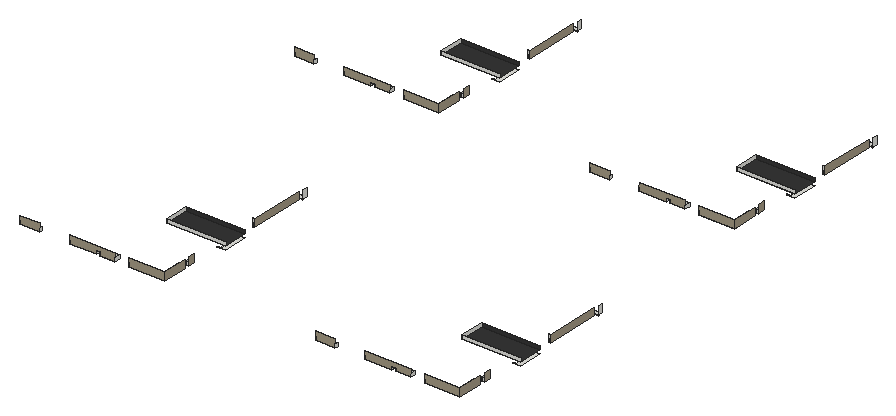
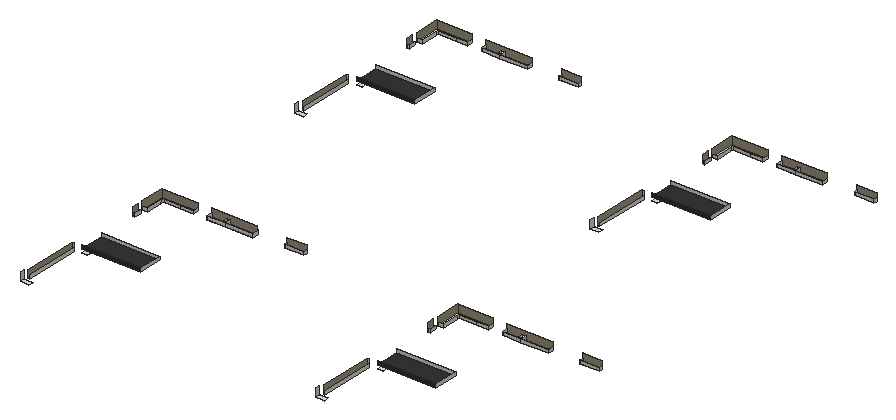
# SketchUp Ruby script. Lengths in inches.
U = 1.inch
M = Sketchup.active_model
def pt(a) = Geom::Point3d.new(a.map { |v| v * U })
def face(e, loops, mat)
  f = e.add_face(loops[0].map { |a| pt(a) })
  loops[1..].each { |l| e.add_face(l.map { |a| pt(a) }).erase! }
  f.material = f.back_material = mat if mat
  f
end
# faces: each face lists its corners as indices into pts; further lists are holes
def faces(e, pts, list, mat = nil) = list.each { |f| face(e, (f[0].is_a?(Array) ? f : [f]).map { |l| l.map { |i| pts[i] } }, mat) }
# xy, xz, yz: faces in a plane at the given z, y or x. An outline is a flat list of corners, or four numbers for a rectangle; further outlines are holes
def ring(l) = l.size == 4 ? [[l[0], l[1]], [l[2], l[1]], [l[2], l[3]], [l[0], l[3]]] : l.each_slice(2).to_a
def flat(e, list, mat, &to3) = list.each { |f| face(e, (f[0].is_a?(Array) ? f : [f]).map { |l| ring(l).map { |u, v| to3.(u, v) } }, mat) }
def xy(e, z, list, mat = nil) = flat(e, list, mat) { |x, y| [x, y, z] }
def xz(e, y, list, mat = nil) = flat(e, list, mat) { |x, z| [x, y, z] }
def yz(e, x, list, mat = nil) = flat(e, list, mat) { |y, z| [x, y, z] }
def lines(e, pts, list) = list.each { |a, b| e.add_line(pt(pts[a]), pt(pts[b])) }
# prism: a flat outline (further loops are holes) pulled along v
def prism(e, loops, v, mat = nil)
  f = face(e, loops, mat); d = Geom::Vector3d.new(v.map { |x| x * U })
  f.pushpull(f.normal.samedirection?(d) ? d.length : -d.length)
end
def box(e, o, s, mat = nil) = prism(e, [[o, [o[0] + s[0], o[1], o[2]], [o[0] + s[0], o[1] + s[1], o[2]], [o[0], o[1] + s[1], o[2]]]], [0, 0, s[2]], mat)
def at(x, y, z, deg = 0) = Geom::Transformation.translation(pt([x, y, z])) * Geom::Transformation.rotation(ORIGIN, Z_AXIS, deg.degrees)
def axes(o, x, y, z) = Geom::Transformation.new([*x, 0, *y, 0, *z, 0, *pt(o).to_a, 1])
def part(name) = M.definitions.add(name)
# library, detail: a bought-in or finely detailed component or shape, given as its bounding box
def library(name, o, s) = part(name).tap { |d| box(d.entities, o, s) }
def detail(e, o, s) = box(e.add_group.entities, o, s)
def put(e, d, t, mat = nil) = e.add_instance(d, t).tap { |i| i.material = mat if mat }
def group(e, t, mat = nil) = e.add_group.tap { |g| g.transformation = t; g.material = mat if mat }.entities
root = M.entities
M.materials.add("[Concrete Tile]").color = [165, 155, 133]
M.materials.add("[Slate Light Tile]").color = [54, 54, 54]
xy(root,88.32,[[879.125,2113.57,879.125,2115.31,892.3125,2115.31,892.3125,2213.62,913.875,2213.62,913.875,2113.57],[2097.3125,2113.57,2097.3125,2115.31,2110.5,2115.31,2110.5,2213.62,2132.0625,2213.62,2132.0625,2113.57],[890.875,2115.31,892.3125,2213.62],[2109.0625,2115.31,2110.5,2213.62],[879.125,3528.25,879.125,3530,892.3125,3530,892.3125,3628.31,913.875,3628.31,913.875,3528.25],
  [2097.3125,3528.25,2097.3125,3530,2110.5,3530,2110.5,3628.31,2132.0625,3628.31,2132.0625,3528.25],[890.875,3530,892.3125,3628.31],[2109.0625,3530,2110.5,3628.31]])
xy(root,103.85,[[671.25,2113.57,913.875,2213.62],[1889.4375,2113.57,2132.0625,2213.62],[671.25,3528.25,913.875,3628.31],[1889.4375,3528.25,2132.0625,3628.31]],"[Slate Light Tile]")
xy(root,112.625,[[319.53,1799.9375,399.88,1811.4375],[521.59,1799.9375,634.11,1822.9375],[647.8,1799.9375,647.8,1814.92,634.11,1814.92,634.11,1822.9375,709.87,1822.9375,709.87,1799.9375],[767.19,1799.9375,767.19,1822.9375,890.875,1822.9375,890.875,1902.66,913.875,1902.66,913.875,1799.9375],[1537.72,1799.9375,1618.07,1811.4375],
  [1739.78,1799.9375,1852.3,1822.9375],[1865.99,1799.9375,1865.99,1814.92,1852.3,1814.92,1852.3,1822.9375,1928.05,1822.9375,1928.05,1799.9375],[1985.38,1799.9375,1985.38,1822.9375,2109.0625,1822.9375,2109.0625,1902.66,2132.0625,1902.66,2132.0625,1799.9375],[902.375,1926.07,913.875,1953.7],[2120.5625,1926.07,2132.0625,1953.7],
  [913.875,2257.8125,921.125,2483.21],[2132.0625,2257.8125,2139.3125,2483.21],[890.875,2497.47,927.0625,2514.84],[2109.0625,2497.47,2145.25,2514.84],[319.53,3214.625,399.88,3226.125],
  [521.59,3214.625,634.11,3237.625],[647.8,3214.625,647.8,3229.61,634.11,3229.61,634.11,3237.625,709.87,3237.625,709.87,3214.625],[767.19,3214.625,767.19,3237.625,890.875,3237.625,890.875,3317.34,913.875,3317.34,913.875,3214.625],[1537.72,3214.625,1618.07,3226.125],[1739.78,3214.625,1852.3,3237.625],
  [1865.99,3214.625,1865.99,3229.61,1852.3,3229.61,1852.3,3237.625,1928.05,3237.625,1928.05,3214.625],[1985.38,3214.625,1985.38,3237.625,2109.0625,3237.625,2109.0625,3317.34,2132.0625,3317.34,2132.0625,3214.625],[902.375,3340.76,913.875,3368.39],[2120.5625,3340.76,2132.0625,3368.39],[913.875,3672.5,921.125,3897.9],
  [2132.0625,3672.5,2139.3125,3897.9],[890.875,3912.16,927.0625,3929.52],[2109.0625,3912.16,2145.25,3929.52]])
xz(root,1799.9375,[[319.53,112.625,399.88,145.375],[521.59,112.625,634.11,112.625,634.11,126,647.8,126,647.8,112.625,709.87,112.625,709.87,145.375,523.04,145.375,523.04,132,521.59,132],[767.19,112.625,913.875,145.375],[1537.72,112.625,1618.07,145.375],[1739.78,112.625,1852.3,112.625,1852.3,126,1865.99,126,1865.99,112.625,1928.05,112.625,1928.05,145.375,1741.23,145.375,1741.23,132,1739.78,132],
  [1985.38,112.625,2132.0625,145.375]],"[Concrete Tile]")
xz(root,1811.4375,[[319.53,112.625,399.88,126],[1537.72,112.625,1618.07,126]])
xz(root,1814.92,[[634.11,112.625,647.8,124.32],[1852.3,112.625,1865.99,124.32]])
xz(root,1822.9375,[[521.59,112.625,634.11,126],[634.11,112.625,709.87,126],[767.19,112.625,817,126],[817,112.625,890.875,126],[1739.78,112.625,1852.3,126],
  [1852.3,112.625,1928.05,126],[1985.38,112.625,2035.1875,126],[2035.1875,112.625,2109.0625,126]])
xz(root,1902.66,[[890.875,112.625,913.875,126],[2109.0625,112.625,2132.0625,126]])
xz(root,1926.07,[[902.375,112.625,913.875,126],[2120.5625,112.625,2132.0625,126]])
xz(root,1953.7,[[902.375,112.625,913.875,126],[2120.5625,112.625,2132.0625,126]])
xz(root,2113.57,[[671.25,103.85,913.875,117.41],[1889.4375,103.85,2132.0625,117.41]])
xz(root,2213.62,[[671.25,103.85,913.875,117.41],[1889.4375,103.85,2132.0625,117.41]],"[Slate Light Tile]")
xz(root,2257.8125,[[913.875,112.625,921.125,143.875],[2132.0625,112.625,2139.3125,143.875]])
xz(root,2497.47,[[921.125,110.625,921.125,112.625,927.0625,112.625,927.0625,143.875,927.75,143.875,927.75,110.625],[2139.3125,110.625,2139.3125,112.625,2145.25,112.625,2145.25,143.875,2145.9375,143.875,2145.9375,110.625]])
xz(root,3214.625,[[319.53,112.625,399.88,145.375],[521.59,112.625,634.11,112.625,634.11,126,647.8,126,647.8,112.625,709.87,112.625,709.87,145.375,523.04,145.375,523.04,132,521.59,132],[767.19,112.625,913.875,145.375],[1537.72,112.625,1618.07,145.375],[1739.78,112.625,1852.3,112.625,1852.3,126,1865.99,126,1865.99,112.625,1928.05,112.625,1928.05,145.375,1741.23,145.375,1741.23,132,1739.78,132],
  [1985.38,112.625,2132.0625,145.375]],"[Concrete Tile]")
xz(root,3226.125,[[319.53,112.625,399.88,126],[1537.72,112.625,1618.07,126]])
xz(root,3229.61,[[634.11,112.625,647.8,124.32],[1852.3,112.625,1865.99,124.32]])
xz(root,3237.625,[[521.59,112.625,634.11,126],[634.11,112.625,709.87,126],[767.19,112.625,817,126],[817,112.625,890.875,126],[1739.78,112.625,1852.3,126],
  [1852.3,112.625,1928.05,126],[1985.38,112.625,2035.1875,126],[2035.1875,112.625,2109.0625,126]])
xz(root,3317.34,[[890.875,112.625,913.875,126],[2109.0625,112.625,2132.0625,126]])
xz(root,3340.76,[[902.375,112.625,913.875,126],[2120.5625,112.625,2132.0625,126]])
xz(root,3368.39,[[902.375,112.625,913.875,126],[2120.5625,112.625,2132.0625,126]])
xz(root,3528.25,[[671.25,103.85,913.875,117.41],[1889.4375,103.85,2132.0625,117.41]])
xz(root,3628.31,[[671.25,103.85,913.875,117.41],[1889.4375,103.85,2132.0625,117.41]],"[Slate Light Tile]")
xz(root,3672.5,[[913.875,112.625,921.125,143.875],[2132.0625,112.625,2139.3125,143.875]])
xz(root,3912.16,[[921.125,110.625,921.125,112.625,927.0625,112.625,927.0625,143.875,927.75,143.875,927.75,110.625],[2139.3125,110.625,2139.3125,112.625,2145.25,112.625,2145.25,143.875,2145.9375,143.875,2145.9375,110.625]])
yz(root,319.53,[[1799.9375,112.625,1811.4375,126],[3214.625,112.625,3226.125,126]])
yz(root,399.88,[[1799.9375,112.625,1811.4375,126],[3214.625,112.625,3226.125,126]])
yz(root,521.59,[[1799.9375,112.625,1822.9375,126],[3214.625,112.625,3237.625,126]])
yz(root,634.11,[[1799.9375,112.625,1814.92,126],[3214.625,112.625,3229.61,126]])
yz(root,647.8,[[1799.9375,112.625,1814.92,126],[3214.625,112.625,3229.61,126]])
yz(root,671.25,[[2113.57,103.85,2213.62,117.41],[3528.25,103.85,3628.31,117.41]])
yz(root,709.87,[[1799.9375,112.625,1822.9375,126],[3214.625,112.625,3237.625,126]])
yz(root,767.19,[[1799.9375,112.625,1822.9375,126],[3214.625,112.625,3237.625,126]])
yz(root,890.875,[[1822.9375,112.625,1834.0625,126],[1834.0625,112.625,1902.66,126],[3237.625,112.625,3248.75,126],[3248.75,112.625,3317.34,126]])
yz(root,902.375,[[1926.07,112.625,1953.7,126],[3340.76,112.625,3368.39,126]])
yz(root,913.875,[[2257.8125,112.625,2483.21,126],[3672.5,112.625,3897.9,126]])
yz(root,913.875,[[1799.9375,112.625,1902.66,145.375],[1926.07,112.625,1953.7,145.375],[3214.625,112.625,3317.34,145.375],[3340.76,112.625,3368.39,145.375]],"[Concrete Tile]")
yz(root,921.125,[[2257.8125,112.625,2483.21,143.875],[3672.5,112.625,3897.9,143.875]],"[Concrete Tile]")
yz(root,927.0625,[[2497.47,112.625,2514.84,145.375],[3912.16,112.625,3929.52,145.375]])
yz(root,1537.72,[[1799.9375,112.625,1811.4375,126],[3214.625,112.625,3226.125,126]])
yz(root,1618.07,[[1799.9375,112.625,1811.4375,126],[3214.625,112.625,3226.125,126]])
yz(root,1739.78,[[1799.9375,112.625,1822.9375,126],[3214.625,112.625,3237.625,126]])
yz(root,1852.3,[[1799.9375,112.625,1814.92,126],[3214.625,112.625,3229.61,126]])
yz(root,1865.99,[[1799.9375,112.625,1814.92,126],[3214.625,112.625,3229.61,126]])
yz(root,1889.4375,[[2113.57,103.85,2213.62,117.41],[3528.25,103.85,3628.31,117.41]])
yz(root,1928.05,[[1799.9375,112.625,1822.9375,126],[3214.625,112.625,3237.625,126]])
yz(root,1985.38,[[1799.9375,112.625,1822.9375,126],[3214.625,112.625,3237.625,126]])
yz(root,2109.0625,[[1822.9375,112.625,1834.0625,126],[1834.0625,112.625,1902.66,126],[3237.625,112.625,3248.75,126],[3248.75,112.625,3317.34,126]])
yz(root,2120.5625,[[1926.07,112.625,1953.7,126],[3340.76,112.625,3368.39,126]])
yz(root,2132.0625,[[2257.8125,112.625,2483.21,126],[3672.5,112.625,3897.9,126]])
yz(root,2132.0625,[[1799.9375,112.625,1902.66,145.375],[1926.07,112.625,1953.7,145.375],[3214.625,112.625,3317.34,145.375],[3340.76,112.625,3368.39,145.375]],"[Concrete Tile]")
yz(root,2139.3125,[[2257.8125,112.625,2483.21,143.875],[3672.5,112.625,3897.9,143.875]],"[Concrete Tile]")
yz(root,2145.25,[[2497.47,112.625,2514.84,145.375],[3912.16,112.625,3929.52,145.375]])
